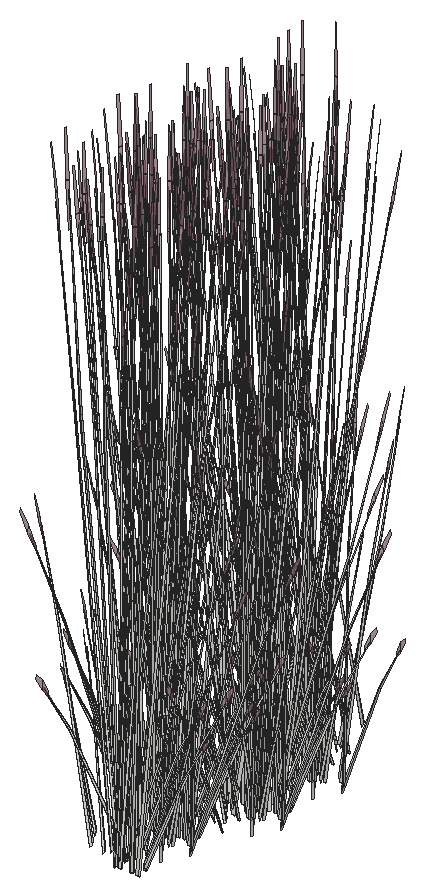
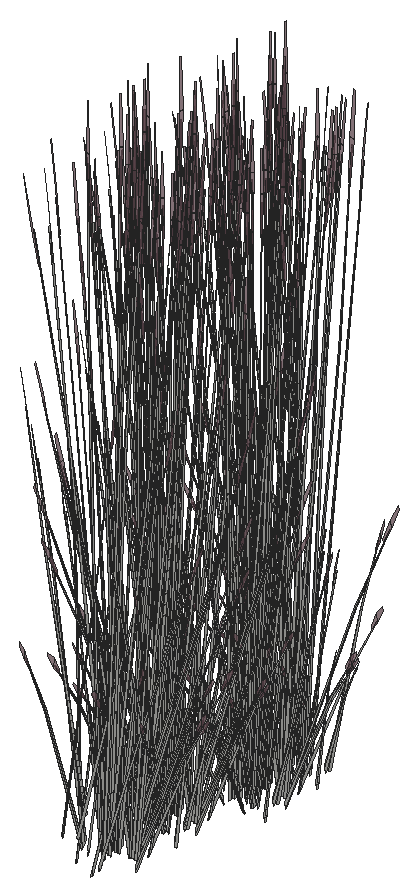
# SketchUp Ruby script. Lengths in inches.
U = 1.inch
M = Sketchup.active_model
def pt(a) = Geom::Point3d.new(a.map { |v| v * U })
def face(e, loops, mat)
  f = e.add_face(loops[0].map { |a| pt(a) })
  loops[1..].each { |l| e.add_face(l.map { |a| pt(a) }).erase! }
  f.material = f.back_material = mat if mat
  f
end
# faces: each face lists its corners as indices into pts; further lists are holes
def faces(e, pts, list, mat = nil) = list.each { |f| face(e, (f[0].is_a?(Array) ? f : [f]).map { |l| l.map { |i| pts[i] } }, mat) }
# xy, xz, yz: faces in a plane at the given z, y or x. An outline is a flat list of corners, or four numbers for a rectangle; further outlines are holes
def ring(l) = l.size == 4 ? [[l[0], l[1]], [l[2], l[1]], [l[2], l[3]], [l[0], l[3]]] : l.each_slice(2).to_a
def flat(e, list, mat, &to3) = list.each { |f| face(e, (f[0].is_a?(Array) ? f : [f]).map { |l| ring(l).map { |u, v| to3.(u, v) } }, mat) }
def xy(e, z, list, mat = nil) = flat(e, list, mat) { |x, y| [x, y, z] }
def xz(e, y, list, mat = nil) = flat(e, list, mat) { |x, z| [x, y, z] }
def yz(e, x, list, mat = nil) = flat(e, list, mat) { |y, z| [x, y, z] }
def lines(e, pts, list) = list.each { |a, b| e.add_line(pt(pts[a]), pt(pts[b])) }
# prism: a flat outline (further loops are holes) pulled along v
def prism(e, loops, v, mat = nil)
  f = face(e, loops, mat); d = Geom::Vector3d.new(v.map { |x| x * U })
  f.pushpull(f.normal.samedirection?(d) ? d.length : -d.length)
end
def box(e, o, s, mat = nil) = prism(e, [[o, [o[0] + s[0], o[1], o[2]], [o[0] + s[0], o[1] + s[1], o[2]], [o[0], o[1] + s[1], o[2]]]], [0, 0, s[2]], mat)
def at(x, y, z, deg = 0) = Geom::Transformation.translation(pt([x, y, z])) * Geom::Transformation.rotation(ORIGIN, Z_AXIS, deg.degrees)
def axes(o, x, y, z) = Geom::Transformation.new([*x, 0, *y, 0, *z, 0, *pt(o).to_a, 1])
def part(name) = M.definitions.add(name)
# library, detail: a bought-in or finely detailed component or shape, given as its bounding box
def library(name, o, s) = part(name).tap { |d| box(d.entities, o, s) }
def detail(e, o, s) = box(e.add_group.entities, o, s)
def put(e, d, t, mat = nil) = e.add_instance(d, t).tap { |i| i.material = mat if mat }
def group(e, t, mat = nil) = e.add_group.tap { |g| g.transformation = t; g.material = mat if mat }.entities
root = M.entities
M.materials.add("LightPink_Translucent").color = [144, 107, 117]
M.materials["LightPink_Translucent"].alpha = 0.75
c1 = part("blade")
p = [[2.15,0.21,22],[0,0.17,0],[0.09,0.45,0],[2.18,0.31,22],[2.29,0.31,22],[0.38,0.45,0],
  [2.48,0.24,33],[2.49,0.24,33],[2.48,0.22,33]]
faces(c1.entities,p,[[0,1,2,3],[4,5,2,3],[6,3,4,7],[8,0,3,6]])
c2 = part("seeds")
p = [[0.3,-0.1,1.38],[-0.01,-0.03,1.59],[-0.01,-0.03,0.03],[0.14,-0.07,-0.07],[0.29,-0.03,3],[0.15,0.01,3.11]]
faces(c2.entities,p,[[0,1,2,3],[1,0,4,5]],"LightPink_Translucent")
c3 = part("blade with seeds")
put(c3.entities,c1,at(0,0,0))
put(c3.entities,c2,axes([2.4,0.25,30.99],[1.5799,-0.05474,1.17369],[-0.12525,1.92788,0.29478],[-0.07173,-0.02425,1.56792]))
put(root,c3,axes([429.53,411.44,152.34],[-0.2532,0.07787,0.97034],[0.11918,-0.32181,0.71294],[0.13432,0.02202,0.21373]))
put(root,c3,axes([426.82,412.37,151.86],[-0.41314,-0.21175,0],[0.19883,-0.43999,0],[0,0,1.37455]))
put(root,c3,axes([427.17,411.8,152.08],[-0.40016,-0.37963,-0.21282],[0.33672,-0.42629,0.46574],[-0.10776,0.04441,1.42109]))
put(root,c3,axes([426.11,412.53,152.09],[0.38354,0.23583,0.41945],[-0.22925,0.42288,0],[-0.08735,-0.05371,1.33059]))
put(root,c3,axes([427.46,410.9,152.3],[0.19883,-0.425,0.37796],[0.41314,0.20454,-0.1819],[0,0.09797,1.2135]))
put(root,c3,axes([427.39,411.14,151.9375],[0,0.54548,-0.04762],[-0.51243,0,0],[0,0.01714,1.5153]))
put(root,c3,axes([425.42,414.36,151.26],[-0.0397,0.06213,1.48974],[-0.40116,0.13396,-0.22758],[-0.09691,-0.12186,0.25375]))
put(root,c3,axes([425.89,412.78,152],[-0.25622,0.47263,0],[-0.42866,-0.26357,-0.43598],[-0.09763,-0.06003,1.38303]))
put(root,c3,axes([428.51,411.13,152.09],[0,-0.47166,0.41945],[0.45849,0,0],[0,0.10742,1.33059]))
put(root,c3,axes([428.33,414.59,151.26],[-0.06134,-0.03716,1.48974],[-0.15755,-0.41512,-0.22758],[0.10629,-0.11265,0.25375]))
put(root,c3,axes([427.36,411.49,152.3],[0.44501,-0.02912,0.37796],[0.04024,0.48332,-0.1819],[-0.07967,0.04899,1.2135]))
put(root,c3,axes([427.64,410.99,152.21],[0.38182,-0.13755,0.12232],[0.13371,0.39278,-0.3493],[0,0.08644,1.07074]))
put(root,c3,axes([429.06,411.95,152.1875],[-0.0987,-0.116,1.20808],[0.12841,-0.38374,-0.25981],[0.19968,0.05198,0.51652]))
put(root,c3,axes([427.29,412.375,151.86],[0.41314,0.21175,0],[-0.19883,0.43999,0],[0,0,1.47801]))
put(root,c3,axes([426.02,414.68,152],[-0.25622,-0.47263,0],[0.42866,-0.26357,-0.43598],[0.09763,-0.06003,1.38303]))
put(root,c3,axes([426.58,414.11,151.8],[-0.28319,0.27058,-0.03288],[-0.25948,-0.29635,-0.1491],[-0.01827,-0.08397,0.4918]))
put(root,c3,axes([427.46,412.84,151.85],[-0.25302,-0.47428,-0.04344],[0.42866,-0.26357,0.43598],[-0.10563,0.04516,1.38235]))
put(root,c3,axes([427.37,411.69,152.21],[0.30276,0.28338,0.12232],[-0.25254,0.31972,-0.3493],[-0.07029,0.04322,1.07074]))
put(root,c3,axes([427.6875,412.57,152.09],[0.38354,-0.23583,0.41945],[0.22925,0.42288,0],[-0.08735,0.05371,1.33059]))
put(root,c3,axes([427.14,412.2,151.9375],[0.17817,0.54185,-0.05079],[-0.50909,0.18987,0],[0.00622,0.01892,1.45452]))
put(root,c3,axes([428.64,415.42,152.1875],[-0.1464,-0.01397,1.20808],[-0.14998,-0.37477,-0.25981],[0.17985,-0.10602,0.51652]))
put(root,c3,axes([424.58,411.95,152.1875],[0.14242,0.03872,1.20808],[0.09179,0.39548,-0.25981],[-0.19345,0.07403,0.51652]))
put(root,c3,axes([428.82,411.21,152.01],[0.51243,0,0],[0,0.52715,-0.43598],[0,0.12006,1.38303]))
put(root,c3,axes([428.61,411.49,151.86],[-0.51218,-0.00377,-0.04204],[0,-0.52715,0.42192],[-0.0161,0.12,1.33776]))
put(root,c3,axes([428.81,414.73,152.34],[-0.1365,0.2401,0.97034],[-0.11733,-0.32258,0.71294],[0.11274,-0.08083,0.21373]))
put(root,c3,axes([427.51,411.03,152.25],[0.46151,0.22505,-0.2458],[-0.22222,0.475,-0.42242],[0.0145,0.11662,1.34921]))
put(root,c3,axes([424.29,412.78,152.34],[0.17079,-0.21377,0.97034],[0.06739,0.33841,0.71294],[-0.12342,0.0606,0.21373]))
put(root,c3,axes([427.28,411.59,152.25],[0.04775,0.53819,-0.2458],[-0.49736,0.03254,-0.42242],[-0.08758,0.07169,1.34921]))
put(root,c3,axes([426.52,415.98,152.25],[-0.04775,-0.53819,-0.2458],[0.49736,-0.03254,-0.42242],[0.08758,-0.07169,1.34921]))
put(root,c3,axes([425.17,414.6,151.8],[-0.11822,0.38513,-0.03288],[-0.36385,-0.11847,-0.1491],[-0.05524,-0.06299,0.4918]))
put(root,c3,axes([426.29,416.55,152.25],[-0.46151,-0.22505,-0.2458],[0.22222,-0.475,-0.42242],[-0.0145,-0.11662,1.34921]))
put(root,c3,axes([424.97,416.36,152],[-0.51243,0,0],[0,-0.52715,-0.43598],[0,-0.12006,1.38303]))
put(root,c3,axes([425.0625,415.42,152.1875],[0.08001,0.13132,1.20808],[-0.18437,0.35694,-0.25981],[-0.18931,-0.08532,0.51652]))
put(root,c3,axes([427.47,412.6,151.97],[0.51304,0.1533,0.25983],[-0.12835,0.54797,-0.30828],[-0.08491,0.06858,1.39295]))
put(root,c3,axes([428.12,412.55,152.34],[-0.23074,-0.13562,0.97034],[0.29794,-0.1378,0.71294],[0.08036,0.11673,0.21373]))
put(root,c3,axes([425.37,416.22,151.97],[-0.38118,0.39654,0.25983],[-0.38142,-0.39237,-0.30828],[-0.01331,-0.11261,1.39295]))
put(root,c3,axes([427.78,412.9,152],[0.25622,0.47263,0],[-0.42866,0.26357,-0.43598],[-0.09763,0.06003,1.38303]))
put(root,c3,axes([428.1875,413.05,151.26],[0.02986,-0.06809,1.48974],[0.37589,-0.20055,-0.22758],[0.11396,0.1038,0.25375]))
put(root,c3,axes([427.56,411.02,152.4],[-0.01119,-0.44408,1.19347],[0.50665,0.11511,0.50532],[-0.11983,0.243,1.12654]))
put(root,c3,axes([424.73,413,151.26],[0.05497,0.04712,1.48974],[0.09321,0.43661,-0.22758],[-0.12183,0.0931,0.25375]))
put(root,c3,axes([426.58,416.4,152.06],[0.46174,0.2286,0.2033],[-0.22222,0.475,0.42242],[0,-0.1095,1.35626]))
put(root,c3,axes([426.4,417.05,152.06],[0.10862,-0.55889,-0.19793],[0.515,0.09742,0.43313],[-0.08999,-0.07718,1.32161]))
put(root,c3,axes([424.59,415.8125,152.34],[0.26163,-0.03375,0.97034],[-0.16596,0.29737,0.71294],[-0.12929,-0.04461,0.21373]))
put(root,c3,axes([428.16,413.17,152.25],[-0.26279,-0.01479,0.88755],[0.17355,-0.31417,0.49003],[0.10382,0.11162,0.6962]))
put(root,c3,axes([426.43,416.09,152.3],[-0.44501,0.02912,0.37796],[-0.04024,-0.48332,-0.1819],[0.07967,-0.04899,1.2135]))
put(root,c3,axes([425.29,416.4375,152.09],[0,0.47166,0.41945],[-0.45849,0,0],[0,-0.10742,1.33059]))
put(root,c3,axes([427.9,414.8,152.01],[0.25622,-0.47263,0],[0.42866,0.26357,-0.43598],[0.09763,0.06003,1.38303]))
put(root,c3,axes([426.42,416.26,151.99],[0.17817,0.52741,0.38653],[-0.50909,0.1834,0.15168],[0.00622,-0.09691,1.34202]))
put(root,c3,axes([428.91,416.66,151.67],[-0.26394,0.0566,1.1961],[-0.04201,-0.45055,0.06846],[0.18486,-0.06819,0.68062]))
put(root,c3,axes([429.39,416.27,151.91],[-0.25407,-0.3016,-0.05481],[0.27826,-0.27635,-0.2485],[0.07884,-0.01946,0.81966]))
put(root,c3,axes([426.33,416.68,152.3],[-0.19883,0.425,0.37796],[-0.41314,-0.20454,-0.1819],[0,-0.09797,1.2135]))
put(root,c3,axes([427.06,416.3,151.86],[0,-0.54574,0],[0.51243,0,0],[0,0,1.51605]))
put(root,c3,axes([427.3,412.41,152.1875],[0.00723,-0.15635,1.20808],[0.34559,-0.17464,-0.25981],[0.10668,0.18713,0.51652]))
put(root,c3,axes([427.68,415.04,152.09],[-0.38354,-0.23583,0.41945],[0.22925,-0.42288,0],[0.08735,0.05371,1.33059]))
put(root,c3,axes([426.82,415.96,151.99],[-0.33979,0.42804,0.38653],[-0.40368,-0.37784,0.15168],[0.08192,-0.04272,1.34202]))
put(root,c3,axes([425.73,413.71,152.34],[-0.01061,-0.28045,0.97034],[0.26501,0.20003,0.71294],[-0.05212,0.13367,0.21373]))
put(root,c3,axes([427.1875,416.73,151.94],[-0.38118,-0.40596,-0.0518],[0.38142,-0.40621,0],[-0.01331,-0.01418,1.48322]))
put(root,c3,axes([426.23,415.26,152.09],[-0.11838,0.46875,0.14904],[-0.43321,-0.13265,0.29641],[0.07483,-0.00228,1.35512]))
put(root,c3,axes([426.43,413.04,151.26],[0.06632,-0.02567,1.48974],[0.39894,0.14126,-0.22758],[0.01167,0.15921,0.25375]))
put(root,c3,axes([426.05,415.63,151.35],[-0.40337,0.18883,1.08919],[-0.12839,-0.54182,0.42321],[0.24769,0.00901,1.23883]))
put(root,c3,axes([427.13,415.78,152.21],[0.07906,-0.42093,0.12232],[0.38625,0.07307,-0.3493],[0.07029,0.04322,1.07074]))
put(root,c3,axes([426.46,416.78,151.99],[0.51796,0.09937,0.38653],[-0.10541,0.56124,0.15168],[-0.07569,-0.05419,1.34202]))
put(root,c3,axes([429.2,416.37,151.26],[-0.02142,-0.07161,1.48974],[0.14855,-0.41887,-0.22758],[0.14984,-0.00603,0.25375]))
put(root,c3,axes([424.78,416.3,151.26],[0.01039,0.07433,1.48974],[-0.20952,0.38819,-0.22758],[-0.14882,-0.01957,0.25375]))
put(root,c3,axes([425.51,413.1,152.38],[0.37228,-0.08352,0.05498],[0.08559,0.3365,-0.7291],[-0.0236,0.17034,0.65354]))
put(root,c3,axes([426.97,415.89,152.3],[-0.24618,-0.39589,0.37796],[0.37289,-0.27878,-0.1819],[0.07967,0.04899,1.2135]))
put(root,c3,axes([426.1875,417.67,152.09],[0.44036,-0.12519,0.14904],[0.10874,0.46588,0.29641],[-0.03927,-0.06788,1.35512]))
put(root,c3,axes([427.09,415.91,152.25],[0.41376,-0.31314,-0.2458],[0.27514,0.44246,-0.42242],[0.10209,0.04493,1.34921]))
put(root,c3,axes([427.41,416.43,151.86],[0.45849,0,0],[0,0.4883,0],[0,0,1.50718]))
put(root,c3,axes([426.63,417.04,152.25],[-0.41376,0.31314,-0.2458],[-0.27514,-0.44246,-0.42242],[-0.10209,-0.04493,1.34921]))
put(root,c3,axes([427.54,415.28,152.09],[-0.44036,0.12519,0.14904],[-0.10874,-0.46588,0.29641],[0.03927,0.06788,1.35512]))
put(root,c3,axes([429.88,420.45,152.1875],[-0.11649,0.09547,1.20808],[-0.34886,-0.1671,-0.25981],[0.06467,-0.20781,0.51652]))
put(root,c3,axes([429.35,420.78,154.21],[-0.19559,-0.38351,-0.60019],[0.40262,-0.21373,0.07243],[-0.04574,-0.1853,0.84903]))
put(root,c3,axes([427.26,416.18,152.01],[-0.51796,-0.09937,0.41563],[0.10541,-0.56124,0.1631],[0.07569,0.05419,1.44303]))
put(root,c3,axes([428.08,420.27,152.1875],[-0.02482,0.15429,1.20808],[-0.36278,0.12916,-0.25981],[-0.0848,-0.19943,0.51652]))
put(root,c3,axes([425.42,413.46,152.1875],[0.12932,-0.07441,1.20808],[0.31929,0.22435,-0.25981],[-0.09503,0.19413,0.51652]))
put(root,c3,axes([426.85,417.5625,151.86],[-0.13371,-0.40664,0],[0.38182,-0.1424,0],[0,0,1.30413]))
put(root,c3,axes([426.59,417.18,152.21],[-0.07906,0.42093,0.12232],[-0.38625,-0.07307,-0.3493],[-0.07029,-0.04322,1.07074]))
put(root,c3,axes([429.02,419.93,151.26],[-0.06874,0.01699,1.48974],[-0.38012,-0.19128,-0.22758],[0.00638,-0.15955,0.25375]))
put(root,c3,axes([427.35,417.51,151.85],[0.43024,-0.16003,-0.16218],[0.15118,0.46099,0.00007],[0.04749,-0.01769,1.46908]))
put(root,c3,axes([427.5,417.7,152.09],[0.11838,-0.46875,0.14904],[0.43321,0.13265,0.29641],[-0.07483,0.00228,1.35512]))
put(root,c3,axes([427.4,416.64,151.87],[0.28606,0.30466,0],[-0.28606,0.30466,0],[0,0,1.42996]))
put(root,c3,axes([430.17,421.16,154.21],[0.01066,-0.43628,-0.60019],[0.44902,0.0293,0.07243],[0.04739,-0.18483,0.84903]))
put(root,c3,axes([428.17,416.5,152.09],[-0.32198,-0.34356,0.14904],[0.32447,-0.33323,0.29641],[-0.03556,0.07016,1.35512]))
put(root,c3,axes([429.46,416.82,152.34],[-0.2532,0.07787,0.97034],[0.11918,-0.32181,0.71294],[0.13432,0.02202,0.21373]))
put(root,c3,axes([426.75,417.75,151.86],[-0.41314,-0.21175,0],[0.19883,-0.43999,0],[0,0,1.37455]))
put(root,c3,axes([427.1,417.18,152.08],[-0.40016,-0.37963,-0.21282],[0.33672,-0.42629,0.46574],[-0.10776,0.04441,1.42109]))
put(root,c3,axes([426.04,417.91,152.09],[0.38354,0.23583,0.41945],[-0.22925,0.42288,0],[-0.08735,-0.05371,1.33059]))
put(root,c3,axes([427.39,416.28,152.3],[0.19883,-0.425,0.37796],[0.41314,0.20454,-0.1819],[0,0.09797,1.2135]))
put(root,c3,axes([429.46,419.69,152.34],[0.05257,0.27504,0.97034],[-0.29163,-0.15233,0.71294],[0.03138,-0.14083,0.21373]))
put(root,c3,axes([427.32,416.52,151.9375],[0,0.54548,-0.04762],[-0.51243,0,0],[0,0.01714,1.5153]))
put(root,c3,axes([425.82,418.16,152],[-0.25622,0.47263,0],[-0.42866,-0.26357,-0.43598],[-0.09763,-0.06003,1.38303]))
put(root,c3,axes([428.4375,416.52,152.09],[0,-0.47166,0.41945],[0.45849,0,0],[0,0.10742,1.33059]))
put(root,c3,axes([427.29,416.87,152.3],[0.44501,-0.02912,0.37796],[0.04024,0.48332,-0.1819],[-0.07967,0.04899,1.2135]))
put(root,c3,axes([427.57,416.375,152.21],[0.38182,-0.13755,0.12232],[0.13371,0.39278,-0.3493],[0,0.08644,1.07074]))
put(root,c3,axes([427.96,420.02,152.34],[0.21377,0.16416,0.97034],[-0.31132,0.09868,0.71294],[-0.06661,-0.12616,0.21373]))
put(root,c3,axes([428.47,420.89,154.21],[-0.34944,-0.22798,-0.60019],[0.24834,-0.39949,0.07243],[-0.1266,-0.13612,0.84903]))
put(root,c3,axes([428.99,417.33,152.1875],[-0.0987,-0.116,1.20808],[0.12841,-0.38374,-0.25981],[0.19968,0.05198,0.51652]))
put(root,c3,axes([427.22,417.76,151.86],[0.41314,0.21175,0],[-0.19883,0.43999,0],[0,0,1.47801]))
put(root,c3,axes([427.39,418.22,151.85],[-0.25302,-0.47428,-0.04344],[0.42866,-0.26357,0.43598],[-0.10563,0.04516,1.38235]))
put(root,c3,axes([427.3,417.08,152.21],[0.30276,0.28338,0.12232],[-0.25254,0.31972,-0.3493],[-0.07029,0.04322,1.07074]))
put(root,c3,axes([427.79,420.52,151.26],[-0.0397,0.06213,1.48974],[-0.40116,0.13396,-0.22758],[-0.09691,-0.12186,0.25375]))
put(root,c3,axes([430.7,420.75,151.26],[-0.06134,-0.03716,1.48974],[-0.15755,-0.41512,-0.22758],[0.10629,-0.11265,0.25375]))
put(root,c3,axes([427.62,417.95,152.09],[0.38354,-0.23583,0.41945],[0.22925,0.42288,0],[-0.08735,0.05371,1.33059]))
put(root,c3,axes([427.07,417.58,151.9375],[0.17817,0.54185,-0.05079],[-0.50909,0.18987,0],[0.00622,0.01892,1.45452]))
put(root,c3,axes([424.51,417.33,152.1875],[0.14242,0.03872,1.20808],[0.09179,0.39548,-0.25981],[-0.19345,0.07403,0.51652]))
put(root,c3,axes([428.75,416.6,152.01],[0.51243,0,0],[0,0.52715,-0.43598],[0,0.12006,1.38303]))
put(root,c3,axes([428.54,416.87,151.86],[-0.51218,-0.00377,-0.04204],[0,-0.52715,0.42192],[-0.0161,0.12,1.33776]))
put(root,c3,axes([427.4375,416.41,152.25],[0.46151,0.22505,-0.2458],[-0.22222,0.475,-0.42242],[0.0145,0.11662,1.34921]))
put(root,c3,axes([430.7,421.92,154.21],[0.21406,-0.37215,-0.60019],[0.37511,0.26448,0.07243],[0.12781,-0.13483,0.84903]))
put(root,c3,axes([428.38,420.83,152],[-0.25622,-0.47263,0],[0.42866,-0.26357,-0.43598],[0.09763,-0.06003,1.38303]))
put(root,c3,axes([424.22,418.16,152.34],[0.17079,-0.21377,0.97034],[0.06739,0.33841,0.71294],[-0.12342,0.0606,0.21373]))
put(root,c3,axes([427.2,416.97,152.25],[0.04775,0.53819,-0.2458],[-0.49736,0.03254,-0.42242],[-0.08758,0.07169,1.34921]))
put(root,c3,axes([428.95,420.26,151.8],[-0.28319,0.27058,-0.03288],[-0.25948,-0.29635,-0.1491],[-0.01827,-0.08397,0.4918]))
put(root,c3,axes([427.4,417.98,151.97],[0.51304,0.1533,0.25983],[-0.12835,0.54797,-0.30828],[-0.08491,0.06858,1.39295]))
put(root,c3,axes([431.01,421.58,152.1875],[-0.1464,-0.01397,1.20808],[-0.14998,-0.37477,-0.25981],[0.17985,-0.10602,0.51652]))
put(root,c3,axes([431.18,420.89,152.34],[-0.1365,0.2401,0.97034],[-0.11733,-0.32258,0.71294],[0.11274,-0.08083,0.21373]))
put(root,c3,axes([428.05,417.93,152.34],[-0.23074,-0.13562,0.97034],[0.29794,-0.1378,0.71294],[0.08036,0.11673,0.21373]))
put(root,c3,axes([428.89,422.14,152.25],[-0.04775,-0.53819,-0.2458],[0.49736,-0.03254,-0.42242],[0.08758,-0.07169,1.34921]))
put(root,c3,axes([427.71,418.28,152],[0.25622,0.47263,0],[-0.42866,0.26357,-0.43598],[-0.09763,0.06003,1.38303]))
put(root,c3,axes([427.54,420.76,151.8],[-0.11822,0.38513,-0.03288],[-0.36385,-0.11847,-0.1491],[-0.05524,-0.06299,0.4918]))
put(root,c3,axes([428.66,422.7,152.25],[-0.46151,-0.22505,-0.2458],[0.22222,-0.475,-0.42242],[-0.0145,-0.11662,1.34921]))
put(root,c3,axes([428.12,418.4375,151.26],[0.02986,-0.06809,1.48974],[0.37589,-0.20055,-0.22758],[0.11396,0.1038,0.25375]))
put(root,c3,axes([427.49,416.41,152.4],[-0.01119,-0.44408,1.19347],[0.50665,0.11511,0.50532],[-0.11983,0.243,1.12654]))
put(root,c3,axes([424.66,418.38,151.26],[0.05497,0.04712,1.48974],[0.09321,0.43661,-0.22758],[-0.12183,0.0931,0.25375]))
put(root,c3,axes([427.34,422.51,152],[-0.51243,0,0],[0,-0.52715,-0.43598],[0,-0.12006,1.38303]))
put(root,c3,axes([427.43,421.57,152.1875],[0.08001,0.13132,1.20808],[-0.18437,0.35694,-0.25981],[-0.18931,-0.08532,0.51652]))
put(root,c3,axes([427.76,421.46,154.21],[-0.40965,-0.01136,-0.60019],[0.02751,-0.47821,0.07243],[-0.17355,-0.05047,0.84903]))
put(root,c3,axes([428.09,418.55,152.25],[-0.26279,-0.01479,0.88755],[0.17355,-0.31417,0.49003],[0.10382,0.11162,0.6962]))
put(root,c3,axes([427.74,422.375,151.97],[-0.38118,0.39654,0.25983],[-0.38142,-0.39237,-0.30828],[-0.01331,-0.11261,1.39295]))
put(root,c3,axes([427.23,417.79,152.1875],[0.00723,-0.15635,1.20808],[0.34559,-0.17464,-0.25981],[0.10668,0.18713,0.51652]))
put(root,c3,axes([428.95,422.56,152.06],[0.46174,0.2286,0.2033],[-0.22222,0.475,0.42242],[0,-0.1095,1.35626]))
put(root,c3,axes([428.77,423.2,152.06],[0.10862,-0.55889,-0.19793],[0.515,0.09742,0.43313],[-0.08999,-0.07718,1.32161]))
put(root,c3,axes([425.66,419.09,152.34],[-0.01061,-0.28045,0.97034],[0.26501,0.20003,0.71294],[-0.05212,0.13367,0.21373]))
put(root,c3,axes([426.95,421.97,152.34],[0.26163,-0.03375,0.97034],[-0.16596,0.29737,0.71294],[-0.12929,-0.04461,0.21373]))
put(root,c3,axes([426.36,418.42,151.26],[0.06632,-0.02567,1.48974],[0.39894,0.14126,-0.22758],[0.01167,0.15921,0.25375]))
put(root,c3,axes([428.8,422.24,152.3],[-0.44501,0.02912,0.37796],[-0.04024,-0.48332,-0.1819],[0.07967,-0.04899,1.2135]))
put(root,c3,axes([427.65,422.59,152.09],[0,0.47166,0.41945],[-0.45849,0,0],[0,-0.10742,1.33059]))
put(root,c3,axes([430.27,420.95,152.01],[0.25622,-0.47263,0],[0.42866,0.26357,-0.43598],[0.09763,0.06003,1.38303]))
put(root,c3,axes([428.79,422.42,151.99],[0.17817,0.52741,0.38653],[-0.50909,0.1834,0.15168],[0.00622,-0.09691,1.34202]))
put(root,c3,axes([425.44,418.49,152.38],[0.37228,-0.08352,0.05498],[0.08559,0.3365,-0.7291],[-0.0236,0.17034,0.65354]))
put(root,c3,axes([431.28,422.82,151.67],[-0.26394,0.0566,1.1961],[-0.04201,-0.45055,0.06846],[0.18486,-0.06819,0.68062]))
put(root,c3,axes([431.76,422.42,151.91],[-0.25407,-0.3016,-0.05481],[0.27826,-0.27635,-0.2485],[0.07884,-0.01946,0.81966]))
put(root,c3,axes([428.7,422.83,152.3],[-0.19883,0.425,0.37796],[-0.41314,-0.20454,-0.1819],[0,-0.09797,1.2135]))
put(root,c3,axes([429.43,422.46,151.86],[0,-0.54574,0],[0.51243,0,0],[0,0,1.51605]))
put(root,c3,axes([430.05,421.2,152.09],[-0.38354,-0.23583,0.41945],[0.22925,-0.42288,0],[0.08735,0.05371,1.33059]))
put(root,c3,axes([430.8,422.86,154.21],[0.3601,-0.20831,-0.60019],[0.20068,0.4288,0.07243],[0.17399,-0.04871,0.84903]))
put(root,c3,axes([429.18,422.12,151.99],[-0.33979,0.42804,0.38653],[-0.40368,-0.37784,0.15168],[0.08192,-0.04272,1.34202]))
put(root,c3,axes([429.56,422.88,151.94],[-0.38118,-0.40596,-0.0518],[0.38142,-0.40621,0],[-0.01331,-0.01418,1.48322]))
put(root,c3,axes([428.59,421.41,152.09],[-0.11838,0.46875,0.14904],[-0.43321,-0.13265,0.29641],[0.07483,-0.00228,1.35512]))
put(root,c3,axes([428.42,421.79,151.35],[-0.40337,0.18883,1.08919],[-0.12839,-0.54182,0.42321],[0.24769,0.00901,1.23883]))
put(root,c3,axes([429.5,421.93,152.21],[0.07906,-0.42093,0.12232],[0.38625,0.07307,-0.3493],[0.07029,0.04322,1.07074]))
put(root,c3,axes([428.83,422.93,151.99],[0.51796,0.09937,0.38653],[-0.10541,0.56124,0.15168],[-0.07569,-0.05419,1.34202]))
put(root,c3,axes([431.57,422.53,151.26],[-0.02142,-0.07161,1.48974],[0.14855,-0.41887,-0.22758],[0.14984,-0.00603,0.25375]))
put(root,c3,axes([427.14,422.45,151.26],[0.01039,0.07433,1.48974],[-0.20952,0.38819,-0.22758],[-0.14882,-0.01957,0.25375]))
put(root,c3,axes([425.35,418.84,152.1875],[0.12932,-0.07441,1.20808],[0.31929,0.22435,-0.25981],[-0.09503,0.19413,0.51652]))
put(root,c3,axes([429.33,422.04,152.3],[-0.24618,-0.39589,0.37796],[0.37289,-0.27878,-0.1819],[0.07967,0.04899,1.2135]))
put(root,c3,axes([428.55,423.83,152.09],[0.44036,-0.12519,0.14904],[0.10874,0.46588,0.29641],[-0.03927,-0.06788,1.35512]))
put(root,c3,axes([429.46,422.07,152.25],[0.41376,-0.31314,-0.2458],[0.27514,0.44246,-0.42242],[0.10209,0.04493,1.34921]))
put(root,c3,axes([429.78,422.58,151.86],[0.45849,0,0],[0,0.4883,0],[0,0,1.50718]))
put(root,c3,axes([429,423.2,152.25],[-0.41376,0.31314,-0.2458],[-0.27514,-0.44246,-0.42242],[-0.10209,-0.04493,1.34921]))
put(root,c3,axes([429.91,421.4375,152.09],[-0.44036,0.12519,0.14904],[-0.10874,-0.46588,0.29641],[0.03927,0.06788,1.35512]))
put(root,c3,axes([429.88,426.5625,152.1875],[-0.11649,0.09547,1.20808],[-0.34886,-0.1671,-0.25981],[0.06467,-0.20781,0.51652]))
put(root,c3,axes([429.35,426.9,154.21],[-0.19559,-0.38351,-0.60019],[0.40262,-0.21373,0.07243],[-0.04574,-0.1853,0.84903]))
put(root,c3,axes([428.08,426.38,152.1875],[-0.02482,0.15429,1.20808],[-0.36278,0.12916,-0.25981],[-0.0848,-0.19943,0.51652]))
put(root,c3,axes([429.63,422.33,152.01],[-0.51796,-0.09937,0.41563],[0.10541,-0.56124,0.1631],[0.07569,0.05419,1.44303]))
put(root,c3,axes([429.21,423.72,151.86],[-0.13371,-0.40664,0],[0.38182,-0.1424,0],[0,0,1.30413]))
put(root,c3,axes([429.02,426.04,151.26],[-0.06874,0.01699,1.48974],[-0.38012,-0.19128,-0.22758],[0.00638,-0.15955,0.25375]))
put(root,c3,axes([428.96,423.33,152.21],[-0.07906,0.42093,0.12232],[-0.38625,-0.07307,-0.3493],[-0.07029,-0.04322,1.07074]))
put(root,c3,axes([429.71,423.66,151.85],[0.43024,-0.16003,-0.16218],[0.15118,0.46099,0.00007],[0.04749,-0.01769,1.46908]))
put(root,c3,axes([429.86,423.86,152.09],[0.11838,-0.46875,0.14904],[0.43321,0.13265,0.29641],[-0.07483,0.00228,1.35512]))
put(root,c3,axes([429.77,422.79,151.87],[0.28606,0.30466,0],[-0.28606,0.30466,0],[0,0,1.42996]))
put(root,c3,axes([430.17,427.27,154.21],[0.01066,-0.43628,-0.60019],[0.44902,0.0293,0.07243],[0.04739,-0.18483,0.84903]))
put(root,c3,axes([430.54,422.66,152.09],[-0.32198,-0.34356,0.14904],[0.32447,-0.33323,0.29641],[-0.03556,0.07016,1.35512]))
put(root,c3,axes([431.83,422.97,152.34],[-0.2532,0.07787,0.97034],[0.11918,-0.32181,0.71294],[0.13432,0.02202,0.21373]))
put(root,c3,axes([429.12,423.9,151.86],[-0.41314,-0.21175,0],[0.19883,-0.43999,0],[0,0,1.37455]))
put(root,c3,axes([429.46,423.34,152.08],[-0.40016,-0.37963,-0.21282],[0.33672,-0.42629,0.46574],[-0.10776,0.04441,1.42109]))
put(root,c3,axes([428.41,424.07,152.09],[0.38354,0.23583,0.41945],[-0.22925,0.42288,0],[-0.08735,-0.05371,1.33059]))
put(root,c3,axes([429.46,425.8,152.34],[0.05257,0.27504,0.97034],[-0.29163,-0.15233,0.71294],[0.03138,-0.14083,0.21373]))
put(root,c3,axes([429.76,422.4375,152.3],[0.19883,-0.425,0.37796],[0.41314,0.20454,-0.1819],[0,0.09797,1.2135]))
put(root,c3,axes([429.68,422.68,151.9375],[0,0.54548,-0.04762],[-0.51243,0,0],[0,0.01714,1.5153]))
put(root,c3,axes([428.1875,424.3125,152],[-0.25622,0.47263,0],[-0.42866,-0.26357,-0.43598],[-0.09763,-0.06003,1.38303]))
put(root,c3,axes([430.8,422.67,152.09],[0,-0.47166,0.41945],[0.45849,0,0],[0,0.10742,1.33059]))
put(root,c3,axes([429.66,423.03,152.3],[0.44501,-0.02912,0.37796],[0.04024,0.48332,-0.1819],[-0.07967,0.04899,1.2135]))
put(root,c3,axes([429.93,422.53,152.21],[0.38182,-0.13755,0.12232],[0.13371,0.39278,-0.3493],[0,0.08644,1.07074]))
put(root,c3,axes([427.96,426.13,152.34],[0.21377,0.16416,0.97034],[-0.31132,0.09868,0.71294],[-0.06661,-0.12616,0.21373]))
put(root,c3,axes([428.47,427,154.21],[-0.34944,-0.22798,-0.60019],[0.24834,-0.39949,0.07243],[-0.1266,-0.13612,0.84903]))
put(root,c3,axes([431.35,423.49,152.1875],[-0.0987,-0.116,1.20808],[0.12841,-0.38374,-0.25981],[0.19968,0.05198,0.51652]))
put(root,c3,axes([429.59,423.91,151.86],[0.41314,0.21175,0],[-0.19883,0.43999,0],[0,0,1.47801]))
put(root,c3,axes([429.75,424.38,151.85],[-0.25302,-0.47428,-0.04344],[0.42866,-0.26357,0.43598],[-0.10563,0.04516,1.38235]))
put(root,c3,axes([429.66,423.23,152.21],[0.30276,0.28338,0.12232],[-0.25254,0.31972,-0.3493],[-0.07029,0.04322,1.07074]))
put(root,c3,axes([427.79,426.63,151.26],[-0.0397,0.06213,1.48974],[-0.40116,0.13396,-0.22758],[-0.09691,-0.12186,0.25375]))
put(root,c3,axes([430.7,426.86,151.26],[-0.06134,-0.03716,1.48974],[-0.15755,-0.41512,-0.22758],[0.10629,-0.11265,0.25375]))
put(root,c3,axes([430.45,423.72,154.21],[0.40965,0.01136,-0.60019],[-0.02751,0.47821,0.07243],[0.17355,0.05047,0.84903]))
put(root,c3,axes([429.99,424.11,152.09],[0.38354,-0.23583,0.41945],[0.22925,0.42288,0],[-0.08735,0.05371,1.33059]))
put(root,c3,axes([429.44,423.73,151.9375],[0.17817,0.54185,-0.05079],[-0.50909,0.18987,0],[0.00622,0.01892,1.45452]))
put(root,c3,axes([426.88,423.49,152.1875],[0.14242,0.03872,1.20808],[0.09179,0.39548,-0.25981],[-0.19345,0.07403,0.51652]))
put(root,c3,axes([431.12,422.75,152.01],[0.51243,0,0],[0,0.52715,-0.43598],[0,0.12006,1.38303]))
put(root,c3,axes([430.91,423.02,151.86],[-0.51218,-0.00377,-0.04204],[0,-0.52715,0.42192],[-0.0161,0.12,1.33776]))
put(root,c3,axes([429.8,422.56,152.25],[0.46151,0.22505,-0.2458],[-0.22222,0.475,-0.42242],[0.0145,0.11662,1.34921]))
put(root,c3,axes([430.7,428.03,154.21],[0.21406,-0.37215,-0.60019],[0.37511,0.26448,0.07243],[0.12781,-0.13483,0.84903]))
put(root,c3,axes([428.38,426.95,152],[-0.25622,-0.47263,0],[0.42866,-0.26357,-0.43598],[0.09763,-0.06003,1.38303]))
put(root,c3,axes([426.58,424.32,152.34],[0.17079,-0.21377,0.97034],[0.06739,0.33841,0.71294],[-0.12342,0.0606,0.21373]))
put(root,c3,axes([428.95,426.375,151.8],[-0.28319,0.27058,-0.03288],[-0.25948,-0.29635,-0.1491],[-0.01827,-0.08397,0.4918]))
put(root,c3,axes([429.57,423.13,152.25],[0.04775,0.53819,-0.2458],[-0.49736,0.03254,-0.42242],[-0.08758,0.07169,1.34921]))
put(root,c3,axes([431.01,427.6875,152.1875],[-0.1464,-0.01397,1.20808],[-0.14998,-0.37477,-0.25981],[0.17985,-0.10602,0.51652]))
put(root,c3,axes([429.76,424.14,151.97],[0.51304,0.1533,0.25983],[-0.12835,0.54797,-0.30828],[-0.08491,0.06858,1.39295]))
put(root,c3,axes([431.18,427,152.34],[-0.1365,0.2401,0.97034],[-0.11733,-0.32258,0.71294],[0.11274,-0.08083,0.21373]))
put(root,c3,axes([430.42,424.09,152.34],[-0.23074,-0.13562,0.97034],[0.29794,-0.1378,0.71294],[0.08036,0.11673,0.21373]))
put(root,c3,axes([428.89,428.25,152.25],[-0.04775,-0.53819,-0.2458],[0.49736,-0.03254,-0.42242],[0.08758,-0.07169,1.34921]))
put(root,c3,axes([430.08,424.43,152],[0.25622,0.47263,0],[-0.42866,0.26357,-0.43598],[-0.09763,0.06003,1.38303]))
put(root,c3,axes([427.54,426.87,151.8],[-0.11822,0.38513,-0.03288],[-0.36385,-0.11847,-0.1491],[-0.05524,-0.06299,0.4918]))
put(root,c3,axes([428.66,428.8125,152.25],[-0.46151,-0.22505,-0.2458],[0.22222,-0.475,-0.42242],[-0.0145,-0.11662,1.34921]))
put(root,c3,axes([430.48,424.59,151.26],[0.02986,-0.06809,1.48974],[0.37589,-0.20055,-0.22758],[0.11396,0.1038,0.25375]))
put(root,c3,axes([427.34,428.625,152],[-0.51243,0,0],[0,-0.52715,-0.43598],[0,-0.12006,1.38303]))
put(root,c3,axes([429.86,422.5625,152.4],[-0.01119,-0.44408,1.19347],[0.50665,0.11511,0.50532],[-0.11983,0.243,1.12654]))
put(root,c3,axes([427.03,424.53,151.26],[0.05497,0.04712,1.48974],[0.09321,0.43661,-0.22758],[-0.12183,0.0931,0.25375]))
put(root,c3,axes([427.43,427.68,152.1875],[0.08001,0.13132,1.20808],[-0.18437,0.35694,-0.25981],[-0.18931,-0.08532,0.51652]))
put(root,c3,axes([427.76,427.57,154.21],[-0.40965,-0.01136,-0.60019],[0.02751,-0.47821,0.07243],[-0.17355,-0.05047,0.84903]))
put(root,c3,axes([430.46,424.71,152.25],[-0.26279,-0.01479,0.88755],[0.17355,-0.31417,0.49003],[0.10382,0.11162,0.6962]))
put(root,c3,axes([427.74,428.49,151.97],[-0.38118,0.39654,0.25983],[-0.38142,-0.39237,-0.30828],[-0.01331,-0.11261,1.39295]))
put(root,c3,axes([429.6,423.94,152.1875],[0.00723,-0.15635,1.20808],[0.34559,-0.17464,-0.25981],[0.10668,0.18713,0.51652]))
put(root,c3,axes([428.95,428.67,152.06],[0.46174,0.2286,0.2033],[-0.22222,0.475,0.42242],[0,-0.1095,1.35626]))
put(root,c3,axes([428.77,429.3125,152.06],[0.10862,-0.55889,-0.19793],[0.515,0.09742,0.43313],[-0.08999,-0.07718,1.32161]))
put(root,c3,axes([426.95,428.08,152.34],[0.26163,-0.03375,0.97034],[-0.16596,0.29737,0.71294],[-0.12929,-0.04461,0.21373]))
put(root,c3,axes([428.03,425.25,152.34],[-0.01061,-0.28045,0.97034],[0.26501,0.20003,0.71294],[-0.05212,0.13367,0.21373]))
put(root,c3,axes([428.8,428.35,152.3],[-0.44501,0.02912,0.37796],[-0.04024,-0.48332,-0.1819],[0.07967,-0.04899,1.2135]))
put(root,c3,axes([427.65,428.71,152.09],[0,0.47166,0.41945],[-0.45849,0,0],[0,-0.10742,1.33059]))
put(root,c3,axes([428.73,424.58,151.26],[0.06632,-0.02567,1.48974],[0.39894,0.14126,-0.22758],[0.01167,0.15921,0.25375]))
put(root,c3,axes([430.27,427.0625,152.01],[0.25622,-0.47263,0],[0.42866,0.26357,-0.43598],[0.09763,0.06003,1.38303]))
put(root,c3,axes([428.79,428.53,151.99],[0.17817,0.52741,0.38653],[-0.50909,0.1834,0.15168],[0.00622,-0.09691,1.34202]))
put(root,c3,axes([427.8125,424.64,152.38],[0.37228,-0.08352,0.05498],[0.08559,0.3365,-0.7291],[-0.0236,0.17034,0.65354]))
put(root,c3,axes([431.28,428.93,151.67],[-0.26394,0.0566,1.1961],[-0.04201,-0.45055,0.06846],[0.18486,-0.06819,0.68062]))
put(root,c3,axes([431.76,428.53,151.91],[-0.25407,-0.3016,-0.05481],[0.27826,-0.27635,-0.2485],[0.07884,-0.01946,0.81966]))
put(root,c3,axes([428.7,428.94,152.3],[-0.19883,0.425,0.37796],[-0.41314,-0.20454,-0.1819],[0,-0.09797,1.2135]))
put(root,c3,axes([429.43,428.57,151.86],[0,-0.54574,0],[0.51243,0,0],[0,0,1.51605]))
put(root,c3,axes([429.88,431.48,152.1875],[-0.11649,0.09547,1.20808],[-0.34886,-0.1671,-0.25981],[0.06467,-0.20781,0.51652]))
put(root,c3,axes([429.35,431.81,154.21],[-0.19559,-0.38351,-0.60019],[0.40262,-0.21373,0.07243],[-0.04574,-0.1853,0.84903]))
put(root,c3,axes([430.05,427.3125,152.09],[-0.38354,-0.23583,0.41945],[0.22925,-0.42288,0],[0.08735,0.05371,1.33059]))
put(root,c3,axes([430.8,428.97,154.21],[0.3601,-0.20831,-0.60019],[0.20068,0.4288,0.07243],[0.17399,-0.04871,0.84903]))
put(root,c3,axes([428.08,431.3,152.1875],[-0.02482,0.15429,1.20808],[-0.36278,0.12916,-0.25981],[-0.0848,-0.19943,0.51652]))
put(root,c3,axes([429.18,428.23,151.99],[-0.33979,0.42804,0.38653],[-0.40368,-0.37784,0.15168],[0.08192,-0.04272,1.34202]))
put(root,c3,axes([429.02,430.96,151.26],[-0.06874,0.01699,1.48974],[-0.38012,-0.19128,-0.22758],[0.00638,-0.15955,0.25375]))
put(root,c3,axes([429.56,429,151.94],[-0.38118,-0.40596,-0.0518],[0.38142,-0.40621,0],[-0.01331,-0.01418,1.48322]))
put(root,c3,axes([428.59,427.52,152.09],[-0.11838,0.46875,0.14904],[-0.43321,-0.13265,0.29641],[0.07483,-0.00228,1.35512]))
put(root,c3,axes([430.17,432.18,154.21],[0.01066,-0.43628,-0.60019],[0.44902,0.0293,0.07243],[0.04739,-0.18483,0.84903]))
put(root,c3,axes([428.42,427.9,151.35],[-0.40337,0.18883,1.08919],[-0.12839,-0.54182,0.42321],[0.24769,0.00901,1.23883]))
put(root,c3,axes([429.5,428.04,152.21],[0.07906,-0.42093,0.12232],[0.38625,0.07307,-0.3493],[0.07029,0.04322,1.07074]))
put(root,c3,axes([428.83,429.04,151.99],[0.51796,0.09937,0.38653],[-0.10541,0.56124,0.15168],[-0.07569,-0.05419,1.34202]))
put(root,c3,axes([431.57,428.64,151.26],[-0.02142,-0.07161,1.48974],[0.14855,-0.41887,-0.22758],[0.14984,-0.00603,0.25375]))
put(root,c3,axes([428.85,424.4,154.21],[0.19559,0.38351,-0.60019],[-0.40262,0.21373,0.07243],[0.04574,0.1853,0.84903]))
put(root,c3,axes([427.14,428.56,151.26],[0.01039,0.07433,1.48974],[-0.20952,0.38819,-0.22758],[-0.14882,-0.01957,0.25375]))
put(root,c3,axes([429.33,428.16,152.3],[-0.24618,-0.39589,0.37796],[0.37289,-0.27878,-0.1819],[0.07967,0.04899,1.2135]))
put(root,c3,axes([427.72,425,152.1875],[0.12932,-0.07441,1.20808],[0.31929,0.22435,-0.25981],[-0.09503,0.19413,0.51652]))
put(root,c3,axes([429.46,430.72,152.34],[0.05257,0.27504,0.97034],[-0.29163,-0.15233,0.71294],[0.03138,-0.14083,0.21373]))
put(root,c3,axes([428.55,429.94,152.09],[0.44036,-0.12519,0.14904],[0.10874,0.46588,0.29641],[-0.03927,-0.06788,1.35512]))
put(root,c3,axes([429.46,428.18,152.25],[0.41376,-0.31314,-0.2458],[0.27514,0.44246,-0.42242],[0.10209,0.04493,1.34921]))
put(root,c3,axes([429.78,428.69,151.86],[0.45849,0,0],[0,0.4883,0],[0,0,1.50718]))
put(root,c3,axes([429,429.31,152.25],[-0.41376,0.31314,-0.2458],[-0.27514,-0.44246,-0.42242],[-0.10209,-0.04493,1.34921]))
